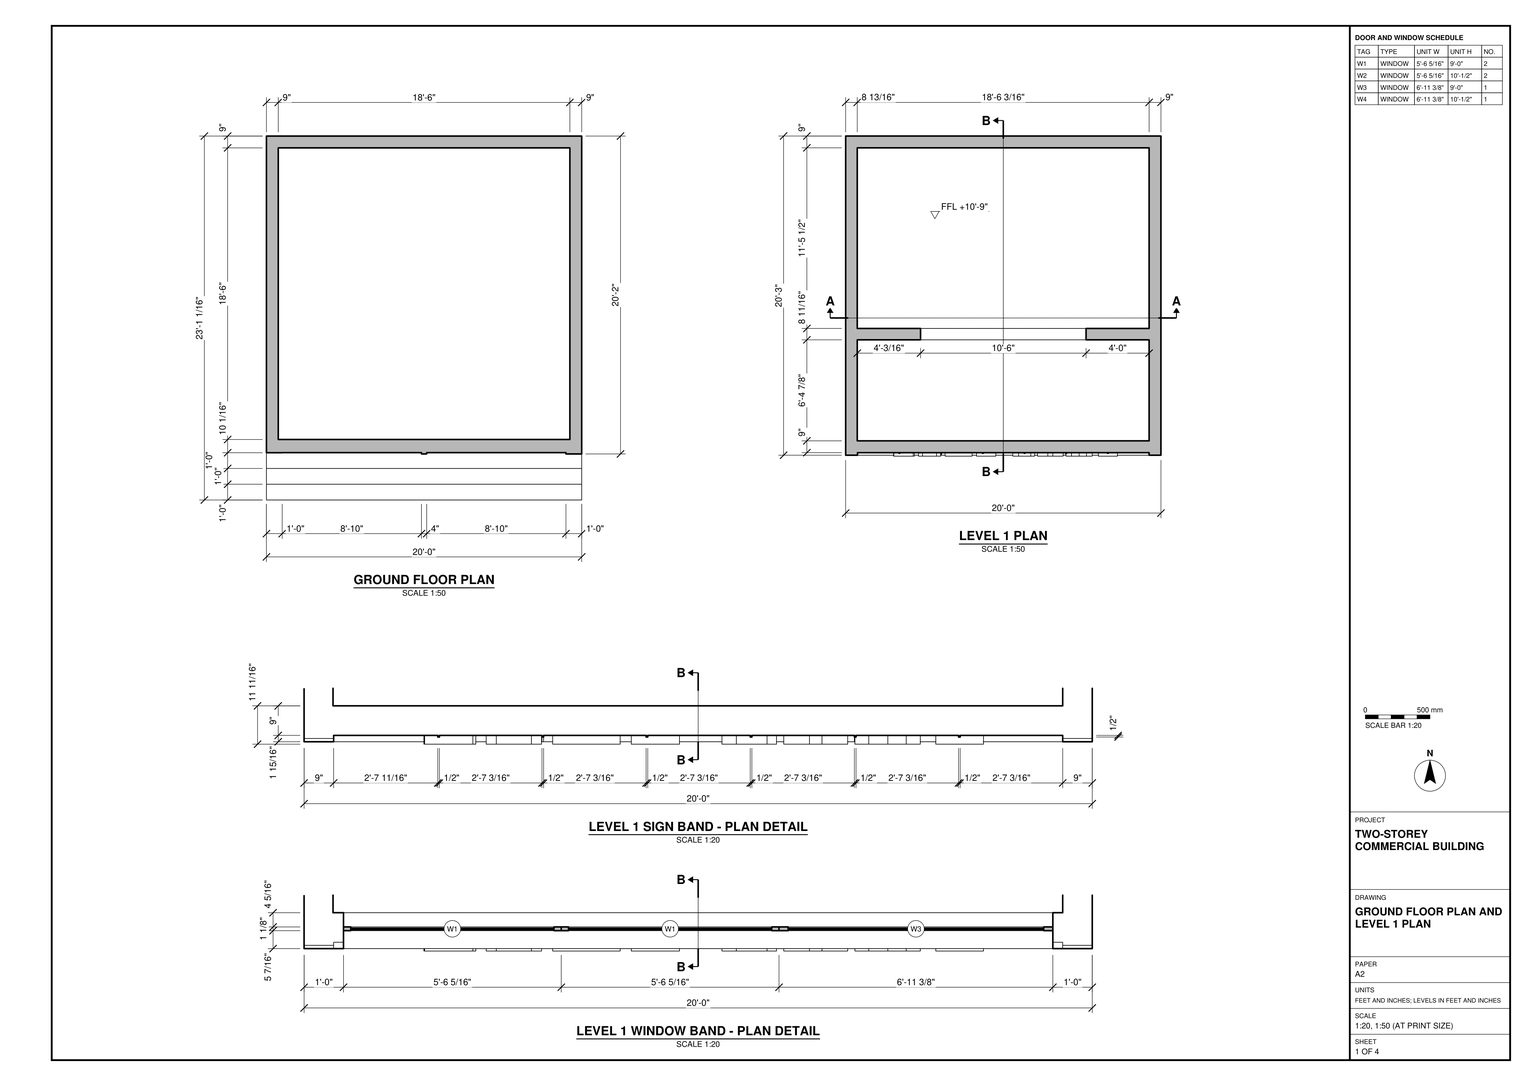
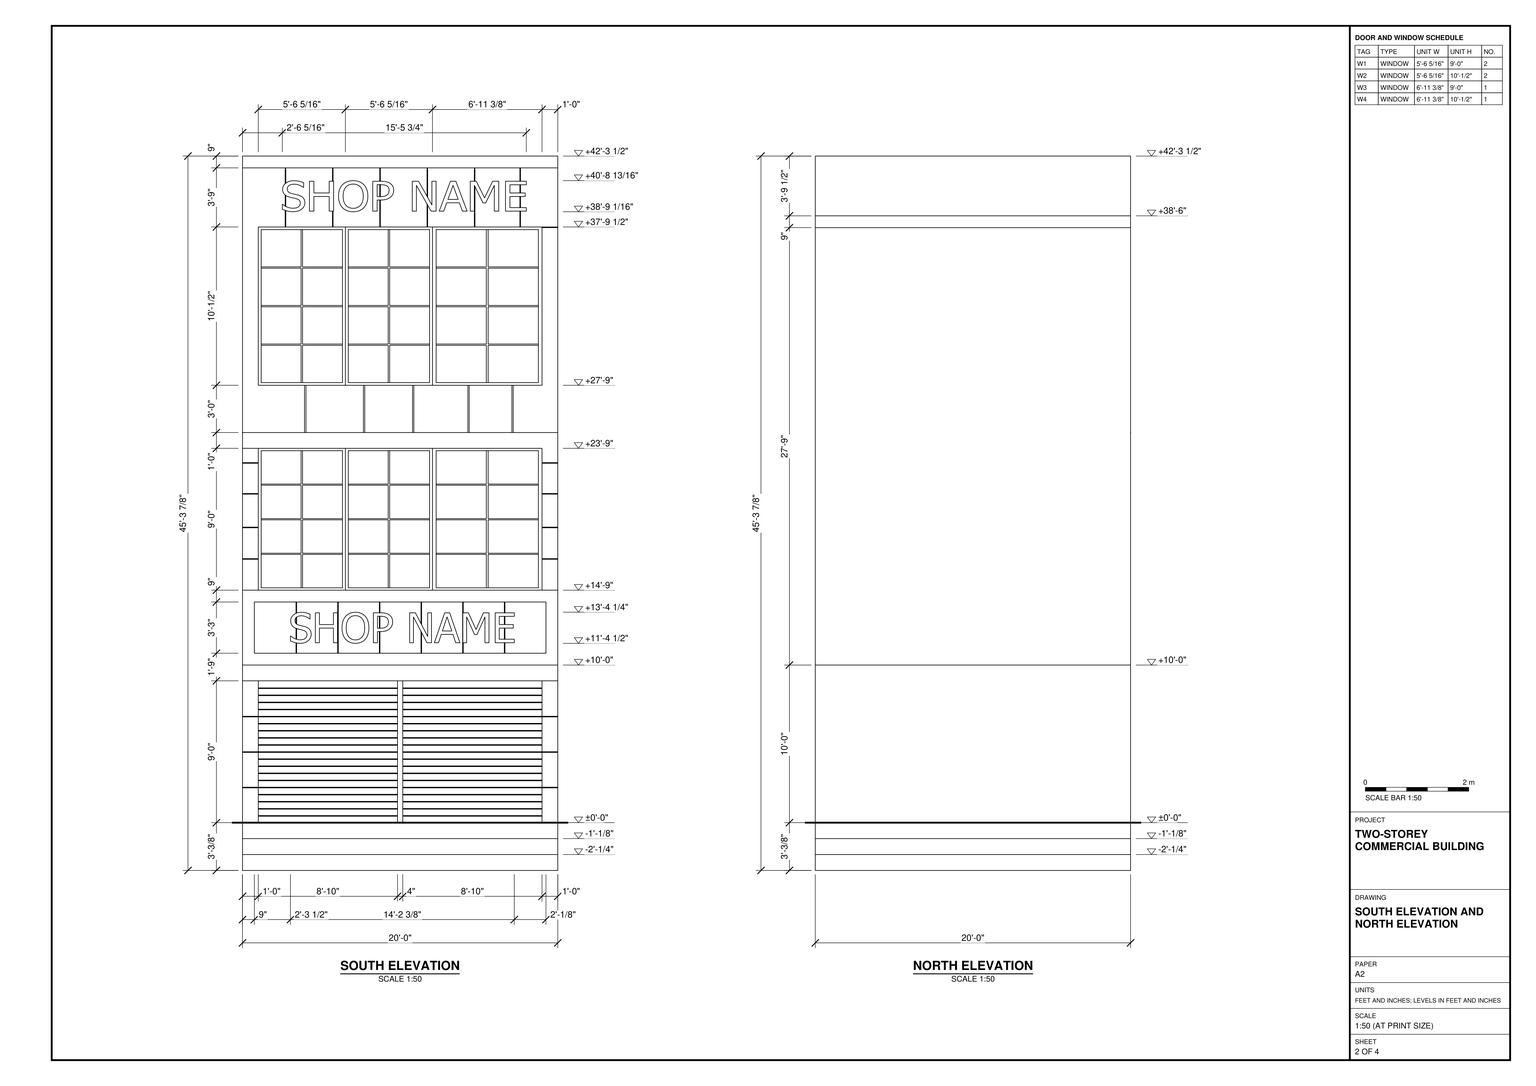
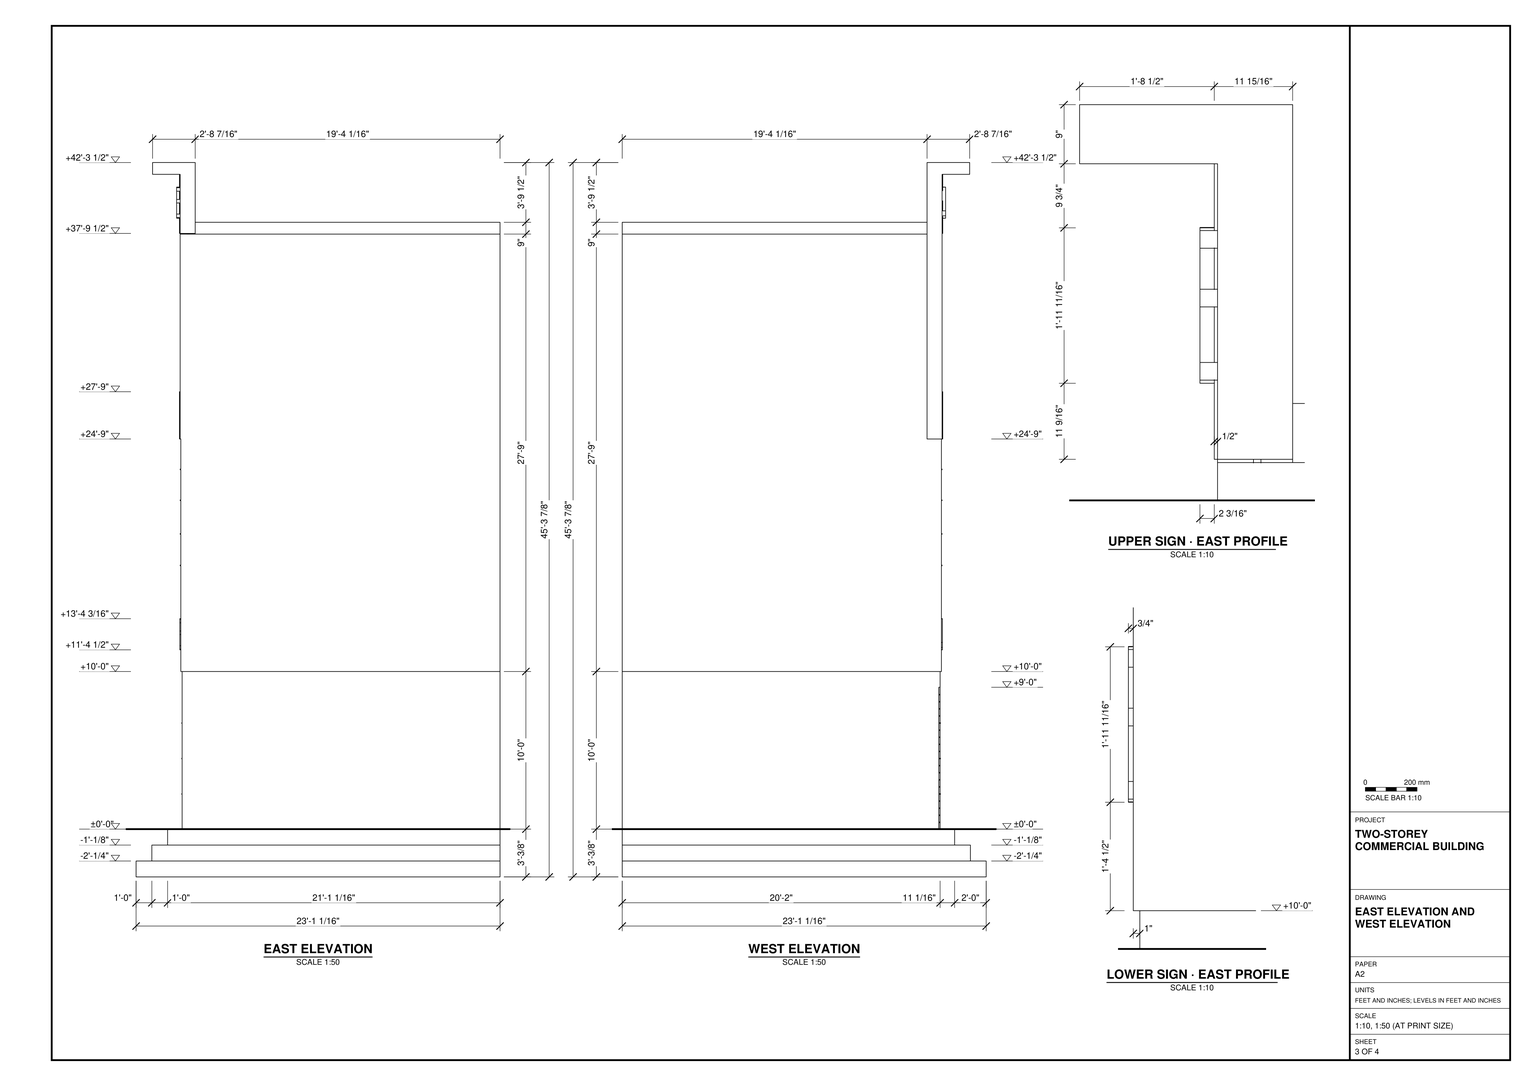
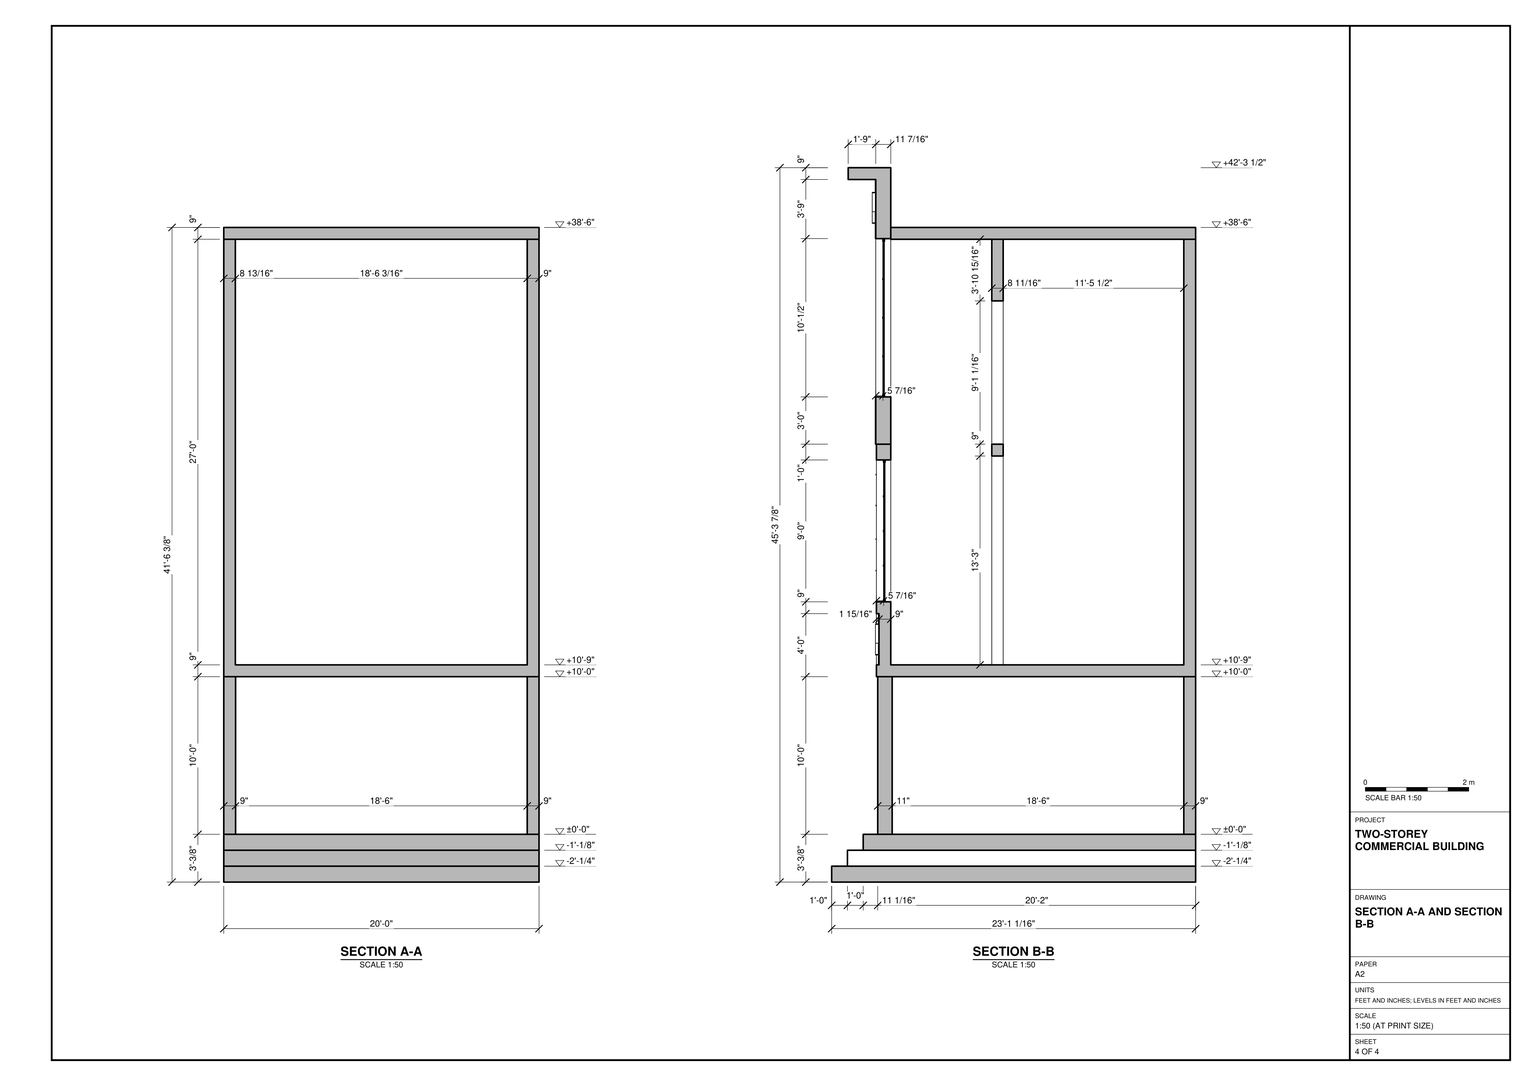
Build the two-storey commercial building in SketchUp from task_files/diagram_01.pdf. Work in feet and inches. Use the south elevation as the shopfront. The overall width is 20'-0", the depth is 23'-1 1/16", and the height is 45'-3 7/8", measured from the bottom of the stepped base to the top of the front cap. Set the ground-floor reference level at ±0'-0" and the level above at +10'-0".

Use the plans to lay out the rectangular shell, with the 9" ground-floor perimeter walls and the wall thicknesses shown on the upper plan. Include the floor slabs, the transverse wall with its broad central opening, and the flat roof slab behind the raised front sign. Keep the side and rear walls plain. Extend the entrance steps across the full shopfront width and model the two horizontally slatted shutter bays with their narrow central pier.

Above the shutters, build the lower sign band, two rows of framed windows separated by a solid band, and the upper sign band with its projecting cap. Follow the window divisions, sign-panel joints and lettering positions in the elevation and detail views.

Keep shell elements and any furniture or joinery pieces in separate groups or components, and use components for repeated parts. Any decor or loose items shown may use suitable library components. Save one SketchUp model as output_files/two_storey_shopfront_with_window_and_sign_bands.skp.

# SketchUp Ruby script. Lengths in inches.
U = 1.inch
M = Sketchup.active_model
def pt(a) = Geom::Point3d.new(a.map { |v| v * U })
def face(e, loops, mat)
  f = e.add_face(loops[0].map { |a| pt(a) })
  loops[1..].each { |l| e.add_face(l.map { |a| pt(a) }).erase! }
  f.material = f.back_material = mat if mat
  f
end
# faces: each face lists its corners as indices into pts; further lists are holes
def faces(e, pts, list, mat = nil) = list.each { |f| face(e, (f[0].is_a?(Array) ? f : [f]).map { |l| l.map { |i| pts[i] } }, mat) }
# xy, xz, yz: faces in a plane at the given z, y or x. An outline is a flat list of corners, or four numbers for a rectangle; further outlines are holes
def ring(l) = l.size == 4 ? [[l[0], l[1]], [l[2], l[1]], [l[2], l[3]], [l[0], l[3]]] : l.each_slice(2).to_a
def flat(e, list, mat, &to3) = list.each { |f| face(e, (f[0].is_a?(Array) ? f : [f]).map { |l| ring(l).map { |u, v| to3.(u, v) } }, mat) }
def xy(e, z, list, mat = nil) = flat(e, list, mat) { |x, y| [x, y, z] }
def xz(e, y, list, mat = nil) = flat(e, list, mat) { |x, z| [x, y, z] }
def yz(e, x, list, mat = nil) = flat(e, list, mat) { |y, z| [x, y, z] }
def lines(e, pts, list) = list.each { |a, b| e.add_line(pt(pts[a]), pt(pts[b])) }
# prism: a flat outline (further loops are holes) pulled along v
def prism(e, loops, v, mat = nil)
  f = face(e, loops, mat); d = Geom::Vector3d.new(v.map { |x| x * U })
  f.pushpull(f.normal.samedirection?(d) ? d.length : -d.length)
end
def box(e, o, s, mat = nil) = prism(e, [[o, [o[0] + s[0], o[1], o[2]], [o[0] + s[0], o[1] + s[1], o[2]], [o[0], o[1] + s[1], o[2]]]], [0, 0, s[2]], mat)
def at(x, y, z, deg = 0) = Geom::Transformation.translation(pt([x, y, z])) * Geom::Transformation.rotation(ORIGIN, Z_AXIS, deg.degrees)
def axes(o, x, y, z) = Geom::Transformation.new([*x, 0, *y, 0, *z, 0, *pt(o).to_a, 1])
def part(name) = M.definitions.add(name)
# library, detail: a bought-in or finely detailed component or shape, given as its bounding box
def library(name, o, s) = part(name).tap { |d| box(d.entities, o, s) }
def detail(e, o, s) = box(e.add_group.entities, o, s)
def put(e, d, t, mat = nil) = e.add_instance(d, t).tap { |i| i.material = mat if mat }
def group(e, t, mat = nil) = e.add_group.tap { |g| g.transformation = t; g.material = mat if mat }.entities
root = M.entities
M.materials.add("[0133_Gray]").color = [128, 128, 128]
M.materials.add("[0134_DimGray]").color = [163, 163, 163]
M.materials.add("[0134_DimGray]1").color = [105, 105, 105]
M.materials.add("[0135_DarkGray]").color = [71, 71, 71]
M.materials.add("[0135_DarkGray]1").color = [81, 81, 81]
M.materials.add("[0136_Charcoal]").color = [73, 73, 73]
M.materials.add("[Blinds Wood Light]").color = [155, 100, 14]
M.materials.add("[Translucent Glass Sky Reflection]").color = [163, 177, 193]
M.materials["[Translucent Glass Sky Reflection]"].alpha = 0.52
M.materials.add("[Wood Cherry Original]").color = [152, 86, 42]
M.materials.add("[Wood Floor Dark]").color = [153, 94, 42]
c1 = library("SHOP NAME",[0.49,0,0],[69.73,9.9,1])
c2 = part("WINDOW")
g1 = group(c2.entities,at(60,0,0))
g2 = group(g1,at(-2,0.5,2),"[Translucent Glass Sky Reflection]")
box(g2,[-56,0,0],[56,0.75,116])
g3 = group(g1,at(0,0,0))
xy(g3,0,[[-60,0,0,2]])
xy(g3,2,[[-58,0,-58,2,-2,2,-2,0,-29.5,0,-29.5,1.25,-30.5,1.25,-30.5,0]])
xy(g3,30.25,[[-58,0,-30.5,1.25],[-29.5,0,-2,1.25]])
xy(g3,31.25,[[-58,0,-30.5,1.25],[-29.5,0,-2,1.25]])
xy(g3,59.5,[[-58,0,-30.5,1.25],[-29.5,0,-2,1.25]])
xy(g3,60.5,[[-58,0,-30.5,1.25],[-29.5,0,-2,1.25]])
xy(g3,88.75,[[-58,0,-30.5,1.25],[-29.5,0,-2,1.25]])
xy(g3,89.75,[[-58,0,-30.5,1.25],[-29.5,0,-2,1.25]])
xy(g3,118,[[-58,0,-30.5,0,-30.5,1.25,-29.5,1.25,-29.5,0,-2,0,-2,2,-58,2]])
xy(g3,120,[[-60,0,0,2]])
xz(g3,0,[[[-60,0,0,120],[-58,2,-30.5,30.25],[-58,31.25,-30.5,59.5],[-29.5,2,-2,30.25],[-58,60.5,-30.5,88.75],[-58,89.75,-30.5,118],[-29.5,89.75,-2,118],[-29.5,60.5,-2,88.75],[-29.5,31.25,-2,59.5]]])
xz(g3,1.25,[[-30.5,2,-29.5,2,-29.5,30.25,-2,30.25,-2,31.25,-29.5,31.25,-29.5,59.5,-2,59.5,-2,60.5,-29.5,60.5,-29.5,88.75,-2,88.75,-2,89.75,-29.5,89.75,-29.5,118,-30.5,118,-30.5,89.75,-58,89.75,-58,88.75,-30.5,88.75,-30.5,60.5,-58,60.5,-58,59.5,-30.5,59.5,-30.5,31.25,-58,31.25,-58,30.25,-30.5,30.25]])
xz(g3,2,[[[-60,0,0,120],[-58,2,-2,118]]])
yz(g3,-60,[[0,0,2,120]])
yz(g3,-58,[[0,2,0,30.25,1.25,30.25,1.25,31.25,0,31.25,0,59.5,1.25,59.5,1.25,60.5,0,60.5,0,88.75,1.25,88.75,1.25,89.75,0,89.75,0,118,2,118,2,2]])
yz(g3,-30.5,[[0,2,1.25,30.25],[0,31.25,1.25,59.5],[0,60.5,1.25,88.75],[0,89.75,1.25,118]])
yz(g3,-29.5,[[0,2,1.25,30.25],[0,31.25,1.25,59.5],[0,60.5,1.25,88.75],[0,89.75,1.25,118]])
yz(g3,-2,[[0,2,2,2,2,118,0,118,0,89.75,1.25,89.75,1.25,88.75,0,88.75,0,60.5,1.25,60.5,1.25,59.5,0,59.5,0,31.25,1.25,31.25,1.25,30.25,0,30.25]])
yz(g3,0,[[0,0,2,120]])
p = [[-29.5,0,118],[-30.5,0,118]]
lines(g3,p,[[0,1]])
xy(root,0,[[[118,35.0625,118,36.0625,12,36.0625,12,36,0,36,0,277.0625,240,277.0625,240,35.0625,228,35.0625,228,36.0625,122,36.0625,122,35.0625],[9,46.0625,231,268.0625]],[9,46.0625,231,268.0625]])
xy(root,4.9,[[12,36.0625,118,37.0625],[122,36.0625,228,37.0625]])
xy(root,5.4,[[12,36.0625,118,37.0625],[122,36.0625,228,37.0625]])
xy(root,10.3,[[12,36.0625,118,37.0625],[122,36.0625,228,37.0625]])
xy(root,10.8,[[12,36.0625,118,37.0625],[122,36.0625,228,37.0625]])
xy(root,15.7,[[12,36.0625,118,37.0625],[122,36.0625,228,37.0625]])
xy(root,16.2,[[12,36.0625,118,37.0625],[122,36.0625,228,37.0625]])
xy(root,21.1,[[12,36.0625,118,37.0625],[122,36.0625,228,37.0625]])
xy(root,21.6,[[12,36.0625,118,37.0625],[122,36.0625,228,37.0625]])
xy(root,26.5,[[228,34.76,240,35.0625],[0,35.7,12,36],[12,36.0625,118,37.0625],[122,36.0625,228,37.0625]])
xy(root,27,[[228,34.76,240,35.0625],[0,35.7,12,36],[12,36.0625,118,37.0625],[122,36.0625,228,37.0625]])
xy(root,31.9,[[12,36.0625,118,37.0625],[122,36.0625,228,37.0625]])
xy(root,32.4,[[12,36.0625,118,37.0625],[122,36.0625,228,37.0625]])
xy(root,37.3,[[12,36.0625,118,37.0625],[122,36.0625,228,37.0625]])
xy(root,37.8,[[12,36,118,37.0625],[122,36.0625,228,37.0625]])
xy(root,42.7,[[12,36,118,37.0625],[122,36.0625,228,37.0625]])
xy(root,43.2,[[12,36.0625,118,37.0625],[122,36.0625,228,37.0625]])
xy(root,48.1,[[12,36.0625,118,37.0625],[122,36.0625,228,37.0625]])
xy(root,48.6,[[12,36.0625,118,37.0625],[122,36.0625,228,37.0625]])
xy(root,53.5,[[228,34.76,240,35.0625],[0,35.7,12,36],[12,36.0625,118,37.0625],[122,36.0625,228,37.0625]])
xy(root,54,[[228,34.76,240,35.0625],[0,35.7,12,36],[12,36.0625,118,37.0625],[122,36.0625,228,37.0625]])
xy(root,58.9,[[12,36.0625,118,37.0625],[122,36.0625,228,37.0625]])
xy(root,59.4,[[12,36.0625,118,37.0625],[122,36.0625,228,37.0625]])
xy(root,64.3,[[12,36.0625,118,37.0625],[122,36.0625,228,37.0625]])
xy(root,64.8,[[12,36.0625,118,37.0625],[122,36.0625,228,37.0625]])
xy(root,69.7,[[12,36.0625,118,37.0625],[122,36.0625,228,37.0625]])
xy(root,70.2,[[12,36.0625,118,37.0625],[122,36.0625,228,37.0625]])
xy(root,75.1,[[12,36.0625,118,37.0625],[122,36.0625,228,37.0625]])
xy(root,75.6,[[12,36.0625,118,37.0625],[122,36.0625,228,37.0625]])
xy(root,80.5,[[228,34.76,240,35.0625],[0,35.7,12,36],[12,36.0625,118,37.0625],[122,36.0625,228,37.0625]])
xy(root,81,[[228,34.76,240,35.0625],[0,35.7,12,36],[12,36.0625,118,37.0625],[122,36.0625,228,37.0625]])
xy(root,85.9,[[12,36.0625,118,37.0625],[122,36.0625,228,37.0625]])
xy(root,86.4,[[12,36.0625,118,37.0625],[122,36.0625,228,37.0625]])
xy(root,91.3,[[12,36.0625,118,37.0625],[122,36.0625,228,37.0625]])
xy(root,91.8,[[12,36.0625,118,37.0625],[122,36.0625,228,37.0625]])
xy(root,96.7,[[12,36.0625,118,37.0625],[122,36.0625,228,37.0625]])
xy(root,97.2,[[12,36.0625,118,37.0625],[122,36.0625,228,37.0625]])
xy(root,102.1,[[12,36.0625,118,37.0625],[122,36.0625,228,37.0625]])
xy(root,102.6,[[12,36.0625,118,37.0625],[122,36.0625,228,37.0625]])
xy(root,108,[[0,35.0625,12,36],[12,35.0625,118,36.0625],[122,35.0625,228,36.0625]])
xy(root,120,[[0,34.0625,240,35.0625],[0,35.0625,240,277.0625]])
xy(root,129,[[9,34.0625,40.71,36],[40.71,34.0625,41.21,35.5],[41.21,34.0625,72.43,36],[72.43,34.0625,72.93,35.5],[72.93,34.0625,104.14,36],
  [104.14,34.0625,104.64,35.5],[104.64,34.0625,135.86,36],[135.86,34.0625,136.36,35.5],[136.36,34.0625,167.57,36],[167.57,34.0625,168.07,35.5],
  [168.07,34.0625,199.29,36],[199.29,34.0625,199.79,35.5],[199.79,34.0625,231,36],[8.8125,45,231,121.9],[57,121.9,183,130.5625],
  [8.8125,130.5625,231,268.0625]])
xy(root,168,[[9,34.0625,40.71,36],[40.71,34.0625,41.21,35.5],[41.21,34.0625,72.43,36],[72.43,34.0625,72.93,35.5],[72.93,34.0625,104.14,36],
  [104.14,34.0625,104.64,35.5],[104.64,34.0625,135.86,36],[135.86,34.0625,136.36,35.5],[136.36,34.0625,167.57,36],[167.57,34.0625,168.07,35.5],
  [168.07,34.0625,199.29,36],[199.29,34.0625,199.79,35.5],[199.79,34.0625,231,36]])
xy(root,177,[[12,34.0625,228,45]])
xy(root,200.5,[[0,33.5625,12,34.0625],[228,33.5625,240,34.0625]])
xy(root,201,[[0,33.5625,12,34.0625],[228,33.5625,240,34.0625]])
xy(root,224.5,[[0,33.5625,12,34.0625],[228,33.5625,240,34.0625]])
xy(root,225,[[0,33.5625,12,34.0625],[228,33.5625,240,34.0625]])
xy(root,250.1,[[0,33.5625,12,34.0625],[228,33.5625,240,34.0625]])
xy(root,250.6,[[0,33.5625,12,34.0625],[228,33.5625,240,34.0625]])
xy(root,273.6,[[0,33.5625,12,34.0625],[228,33.5625,240,34.0625]])
xy(root,274.1,[[0,33.5625,12,34.0625],[228,33.5625,240,34.0625]])
xy(root,285,[[12,34.0625,228,45]])
xy(root,288,[[9,121.9,183,130.5625]])
xy(root,297,[[47.1875,33.0625,48.3125,34.0625],[92.0625,33.0625,93.0625,34.0625],[129.4375,33.0625,130.4375,34.0625],[171.5625,33.0625,172.5625,34.0625],[205.0625,33.0625,206.0625,34.0625],
  [0,33.5625,47.1875,34.0625],[48.3125,33.5625,92.0625,34.0625],[93.0625,33.5625,129.4375,34.0625],[130.4375,33.5625,171.5625,34.0625],[172.5625,33.5625,205.0625,34.0625],
  [206.0625,33.5625,231,34.0625],[231,33.5625,240,34.0625],[0,34.0625,231,45],[8.8125,121.9,9,130.5625],[57,121.9,183,130.5625]])
xy(root,333,[[47.1875,33.0625,48.3125,33.0625,48.3125,33.5625,92.0625,33.5625,92.0625,33.0625,93.0625,33.0625,93.0625,33.5625,129.4375,33.5625,129.4375,33.0625,130.4375,33.0625,130.4375,33.5625,171.5625,33.5625,171.5625,33.0625,172.5625,33.0625,172.5625,33.5625,205.0625,33.5625,205.0625,33.0625,206.0625,33.0625,206.0625,33.5625,228,33.5625,228,45,12,45,12,33.5625,47.1875,33.5625]])
xy(root,406.07,[[57,121.9,183,130.5625]])
xy(root,453,[[228,33.5625,240,45],[0,45,8.8125,277.0625],[8.8125,45,231,268.0625],[231,45,240,277.0625],[9,121.9,57,130.5625],
  [57,121.9,231,130.5625],[8.8125,268.0625,231,277.0625]])
xy(root,453.5,[[32.46,33.0625,32.46,33.5625,12,33.5625,12,45,240,45,240,33.5625,211.65,33.5625,211.65,33.0625,211.15,33.0625,211.15,33.5625,176.96,33.5625,176.96,33.0625,176.46,33.0625,176.46,33.5625,140.96,33.5625,140.96,33.0625,140.46,33.0625,140.46,33.5625,104.96,33.5625,104.96,33.0625,104.46,33.0625,104.46,33.5625,68.96,33.5625,68.96,33.0625,68.45,33.0625,68.45,33.5625,32.96,33.5625,32.96,33.0625]])
xy(root,462,[[0,45,240,277.0625]])
xy(root,498.5,[[0,12.5625,0,33.5625,32.46,33.5625,32.46,33.0625,32.96,33.0625,32.96,33.5625,68.45,33.5625,68.45,33.0625,68.96,33.0625,68.96,33.5625,104.46,33.5625,104.46,33.0625,104.96,33.0625,104.96,33.5625,140.46,33.5625,140.46,33.0625,140.96,33.0625,140.96,33.5625,176.46,33.5625,176.46,33.0625,176.96,33.0625,176.96,33.5625,211.15,33.5625,211.15,33.0625,211.65,33.0625,211.65,33.5625,240,33.5625,240,12.5625]],"[Wood Cherry Original]")
xy(root,507.5,[[0,12.5625,240,45]])
xz(root,12.5625,[[0,498.5,240,507.5]],"[0134_DimGray]1")
xz(root,33.0625,[[47.1875,297,48.3125,333],[92.0625,297,93.0625,333],[129.4375,297,130.4375,333],[171.5625,297,172.5625,333],[205.0625,297,206.0625,333],
  [32.46,453.5,32.96,498.5],[68.45,453.5,68.96,498.5],[104.46,453.5,104.96,498.5],[140.46,453.5,140.96,498.5],[176.46,453.5,176.96,498.5],
  [211.15,453.5,211.65,498.5]],"[0135_DarkGray]1")
xz(root,33.5625,[[228,200.5,240,201],[228,224.5,240,225],[228,250.1,240,250.6],[228,273.6,240,274.1],[140.46,498.5,140.96,507.5]])
xz(root,33.5625,[[0,297,47.1875,297,47.1875,333,12,333,12,453.5,32.46,453.5,32.46,498.5,0,498.5],[48.3125,297,92.0625,333],[93.0625,297,129.4375,333],[130.4375,297,171.5625,333],[172.5625,297,205.0625,333],
  [206.0625,297,240,297,240,453,228,453,228,333,206.0625,333],[32.96,453.5,68.45,498.5],[68.96,453.5,104.46,498.5],[104.96,453.5,140.46,498.5],[140.96,453.5,176.46,498.5],
  [176.96,453.5,211.15,498.5],[211.65,453.5,240,498.5]],"[0133_Gray]")
xz(root,33.5625,[[0,200.5,12,201],[0,224.5,12,225],[0,250.1,12,250.6],[0,273.6,12,274.1]],"[0135_DarkGray]1")
xz(root,34.0625,[[[0,120,240,177],[9,129,231,168]]])
xz(root,34.0625,[[0,177,12,200.5],[0,201,12,224.5],[0,225,12,250.1],[0,250.6,12,273.6],[0,274.1,12,285]],"[0133_Gray]")
xz(root,34.0625,[[228,177,240,200.5],[228,201,240,224.5],[228,225,240,250.1],[228,250.6,240,273.6],[228,274.1,240,274.1,240,297,0,297,0,285,228,285]],"[Wood Floor Dark]")
xz(root,34.76,[[228,26.5,240,27],[228,53.5,240,54],[228,80.5,240,81]],"[0134_DimGray]")
xz(root,35.0625,[[118,0,122,108],[228,0,240,26.5],[228,27,240,53.5],[228,54,240,80.5],[228,81,240,108]],"[0135_DarkGray]")
xz(root,35.0625,[[0,108,240,120]],"[Wood Floor Dark]")
xz(root,35.5,[[40.71,129,41.21,168],[72.43,129,72.93,168],[104.14,129,104.64,168],[135.86,129,136.36,168],[167.57,129,168.07,168],
  [199.29,129,199.79,168]],"[0133_Gray]")
xz(root,35.7,[[0,26.5,12,27],[0,53.5,12,54],[0,80.5,12,81]],"[0134_DimGray]")
xz(root,36,[[12,37.8,118,42.7]],"[0133_Gray]")
xz(root,36,[[0,0,12,26.5],[0,27,12,53.5],[0,54,12,80.5],[0,81,12,108],[9,129,40.71,168],
  [41.21,129,72.43,168],[72.93,129,104.14,168],[104.64,129,135.86,168],[136.36,129,167.57,168],[168.07,129,199.29,168],
  [199.79,129,231,168]],"[0135_DarkGray]")
xz(root,36.0625,[[12,0,118,4.9],[122,0,228,4.9],[12,5.4,118,10.3],[122,5.4,228,10.3],[12,10.8,118,15.7],
  [122,10.8,228,15.7],[12,16.2,118,21.1],[122,16.2,228,21.1],[12,21.6,118,26.5],[122,21.6,228,26.5],
  [12,27,118,31.9],[122,27,228,31.9],[12,32.4,118,37.3],[122,32.4,228,37.3],[122,37.8,228,42.7],
  [12,43.2,118,48.1],[122,43.2,228,48.1],[12,48.6,118,53.5],[122,48.6,228,53.5],[12,54,118,58.9],
  [122,54,228,58.9],[12,59.4,118,64.3],[122,59.4,228,64.3],[12,64.8,118,69.7],[122,64.8,228,69.7],
  [12,70.2,118,75.1],[122,70.2,228,75.1],[12,75.6,118,80.5],[122,75.6,228,80.5],[12,81,118,85.9],
  [122,81,228,85.9],[12,86.4,118,91.3],[122,86.4,228,91.3],[12,91.8,118,96.7],[122,91.8,228,96.7],
  [12,97.2,118,102.1],[122,97.2,228,102.1],[12,102.6,118,108],[122,102.6,228,108]],"[0133_Gray]")
xz(root,37.0625,[[12,4.9,118,5.4],[122,4.9,228,5.4],[12,10.3,118,10.8],[122,10.3,228,10.8],[12,15.7,118,16.2],
  [122,15.7,228,16.2],[12,21.1,118,21.6],[122,21.1,228,21.6],[12,26.5,118,27],[122,26.5,228,27],
  [12,31.9,118,32.4],[122,31.9,228,32.4],[12,37.3,118,37.8],[122,37.3,228,37.8],[12,42.7,118,43.2],
  [122,42.7,228,43.2],[12,48.1,118,48.6],[122,48.1,228,48.6],[12,53.5,118,54],[122,53.5,228,54],
  [12,58.9,118,59.4],[122,58.9,228,59.4],[12,64.3,118,64.8],[122,64.3,228,64.8],[12,69.7,118,70.2],
  [122,69.7,228,70.2],[12,75.1,118,75.6],[122,75.1,228,75.6],[12,80.5,118,81],[122,80.5,228,81],
  [12,85.9,118,86.4],[122,85.9,228,86.4],[12,91.3,118,91.8],[122,91.3,228,91.8],[12,96.7,118,97.2],
  [122,96.7,228,97.2],[12,102.1,118,102.6],[122,102.1,228,102.6]],"[0136_Charcoal]")
xz(root,45,[[8.8125,129,8.8125,297,231,297,231,285,12,285,12,177,231,177,231,129],[228,177,231,285],[0,297,8.8125,453],[8.8125,297,8.8125,453,12,453,12,333,228,333,228,453,231,453,231,297],[0,453,0,462,240,462,240,453.5,12,453.5,12,453],
  [12,453,240,453.5],[0,462,240,507.5]])
xz(root,46.0625,[[9,0,231,120]])
xz(root,121.9,[[8.8125,129,57,288],[183,129,231,129,231,453,57,453,57,406.07,183,406.07],[8.8125,288,9,297],[9,288,57,453],[57,288,183,297]])
xz(root,130.5625,[[8.8125,129,57,288],[183,129,183,288,57,288,57,297,183,297,183,406.07,57,406.07,57,453,231,453,231,129],[8.8125,288,9,297],[9,288,57,453]])
xz(root,268.0625,[[9,0,231,120],[8.8125,129,231,453]])
xz(root,277.0625,[[0,0,240,120],[0,120,240,453],[0,453,240,462]])
yz(root,0,[[36,0,36,26.5,35.7,26.5,35.7,27,36,27,36,53.5,35.7,53.5,35.7,54,36,54,36,80.5,35.7,80.5,35.7,81,36,81,36,108,35.0625,108,35.0625,120,277.0625,120,277.0625,0],[34.0625,120,34.0625,200.5,33.5625,200.5,33.5625,201,34.0625,201,34.0625,224.5,33.5625,224.5,33.5625,225,34.0625,225,34.0625,250.1,33.5625,250.1,33.5625,250.6,34.0625,250.6,34.0625,273.6,33.5625,273.6,33.5625,274.1,34.0625,274.1,34.0625,297,45,297,45,453,277.0625,453,277.0625,120],[33.5625,297,33.5625,498.5,12.5625,498.5,12.5625,507.5,45,507.5,45,297],[45,453,277.0625,462]])
yz(root,8.8125,[[45,129,121.9,129,121.9,297,130.5625,297,130.5625,129,268.0625,129,268.0625,453,45,453]])
yz(root,9,[[46.0625,0,268.0625,120],[34.0625,129,36,168],[121.9,288,130.5625,297],[121.9,297,130.5625,453]])
yz(root,12,[[36,0,36.0625,4.9],[36,4.9,37.0625,5.4],[36,5.4,36.0625,10.3],[36,10.3,37.0625,10.8],[36,10.8,36.0625,15.7],
  [36,15.7,37.0625,16.2],[36,16.2,36.0625,21.1],[36,21.1,37.0625,21.6],[36,21.6,36.0625,26.5],[35.7,26.5,37.0625,27],
  [36,27,36.0625,31.9],[36,31.9,37.0625,32.4],[36,32.4,36.0625,37.3],[36,37.3,37.0625,37.8],[36,42.7,37.0625,43.2],
  [36,43.2,36.0625,48.1],[36,48.1,37.0625,48.6],[36,48.6,36.0625,53.5],[35.7,53.5,37.0625,54],[36,54,36.0625,58.9],
  [36,58.9,37.0625,59.4],[36,59.4,36.0625,64.3],[36,64.3,37.0625,64.8],[36,64.8,36.0625,69.7],[36,69.7,37.0625,70.2],
  [36,70.2,36.0625,75.1],[36,75.1,37.0625,75.6],[36,75.6,36.0625,80.5],[35.7,80.5,37.0625,81],[36,81,36.0625,85.9],
  [36,85.9,37.0625,86.4],[36,86.4,36.0625,91.3],[36,91.3,37.0625,91.8],[36,91.8,36.0625,96.7],[36,96.7,37.0625,97.2],
  [36,97.2,36.0625,102.1],[36,102.1,37.0625,102.6],[36,102.6,36.0625,108],[34.0625,177,45,177,45,285,34.0625,285,34.0625,274.1,33.5625,274.1,33.5625,273.6,34.0625,273.6,34.0625,250.6,33.5625,250.6,33.5625,250.1,34.0625,250.1,34.0625,225,33.5625,225,33.5625,224.5,34.0625,224.5,34.0625,201,33.5625,201,33.5625,200.5,34.0625,200.5],[33.5625,333,45,453.5]])
yz(root,32.46,[[33.0625,453.5,33.5625,498.5]])
yz(root,32.96,[[33.0625,453.5,33.5625,498.5]])
yz(root,40.71,[[35.5,129,36,168]])
yz(root,41.21,[[35.5,129,36,168]])
yz(root,47.1875,[[33.0625,297,33.5625,333]])
yz(root,48.3125,[[33.0625,297,33.5625,333]])
yz(root,57,[[121.9,129,130.5625,297],[121.9,297,130.5625,406.07]])
yz(root,68.45,[[33.0625,453.5,33.5625,498.5]])
yz(root,68.96,[[33.0625,453.5,33.5625,498.5]])
yz(root,72.43,[[35.5,129,36,168]])
yz(root,72.93,[[35.5,129,36,168]])
yz(root,92.0625,[[33.0625,297,33.5625,333]])
yz(root,93.0625,[[33.0625,297,33.5625,333]])
yz(root,104.14,[[35.5,129,36,168]])
yz(root,104.46,[[33.0625,453.5,33.5625,498.5]])
yz(root,104.64,[[35.5,129,36,168]])
yz(root,104.96,[[33.0625,453.5,33.5625,498.5]])
yz(root,118,[[35.0625,4.9,37.0625,5.4],[35.0625,10.3,37.0625,10.8],[35.0625,15.7,37.0625,16.2],[35.0625,21.1,37.0625,21.6],[35.0625,26.5,37.0625,27],
  [35.0625,31.9,37.0625,32.4],[35.0625,37.3,37.0625,37.8],[35.0625,42.7,37.0625,43.2],[35.0625,48.1,37.0625,48.6],[35.0625,53.5,37.0625,54],
  [35.0625,58.9,37.0625,59.4],[35.0625,64.3,37.0625,64.8],[35.0625,69.7,37.0625,70.2],[35.0625,75.1,37.0625,75.6],[35.0625,80.5,37.0625,81],
  [35.0625,85.9,37.0625,86.4],[35.0625,91.3,37.0625,91.8],[35.0625,96.7,37.0625,97.2],[35.0625,102.1,37.0625,102.6]])
yz(root,118,[[35.0625,0,36.0625,4.9],[35.0625,5.4,36.0625,10.3],[35.0625,10.8,36.0625,15.7],[35.0625,16.2,36.0625,21.1],[35.0625,21.6,36.0625,26.5],
  [35.0625,27,36.0625,31.9],[35.0625,32.4,36.0625,37.3],[35.0625,37.8,36,42.7],[35.0625,43.2,36.0625,48.1],[35.0625,48.6,36.0625,53.5],
  [35.0625,54,36.0625,58.9],[35.0625,59.4,36.0625,64.3],[35.0625,64.8,36.0625,69.7],[35.0625,70.2,36.0625,75.1],[35.0625,75.6,36.0625,80.5],
  [35.0625,81,36.0625,85.9],[35.0625,86.4,36.0625,91.3],[35.0625,91.8,36.0625,96.7],[35.0625,97.2,36.0625,102.1],[35.0625,102.6,36.0625,108]],"[0135_DarkGray]")
yz(root,122,[[35.0625,4.9,37.0625,5.4],[35.0625,10.3,37.0625,10.8],[35.0625,15.7,37.0625,16.2],[35.0625,21.1,37.0625,21.6],[35.0625,26.5,37.0625,27],
  [35.0625,31.9,37.0625,32.4],[35.0625,37.3,37.0625,37.8],[35.0625,42.7,37.0625,43.2],[35.0625,48.1,37.0625,48.6],[35.0625,53.5,37.0625,54],
  [35.0625,58.9,37.0625,59.4],[35.0625,64.3,37.0625,64.8],[35.0625,69.7,37.0625,70.2],[35.0625,75.1,37.0625,75.6],[35.0625,80.5,37.0625,81],
  [35.0625,85.9,37.0625,86.4],[35.0625,91.3,37.0625,91.8],[35.0625,96.7,37.0625,97.2],[35.0625,102.1,37.0625,102.6]])
yz(root,122,[[35.0625,0,36.0625,4.9],[35.0625,5.4,36.0625,10.3],[35.0625,10.8,36.0625,15.7],[35.0625,16.2,36.0625,21.1],[35.0625,21.6,36.0625,26.5],
  [35.0625,27,36.0625,31.9],[35.0625,32.4,36.0625,37.3],[35.0625,37.8,36.0625,42.7],[35.0625,43.2,36.0625,48.1],[35.0625,48.6,36.0625,53.5],
  [35.0625,54,36.0625,58.9],[35.0625,59.4,36.0625,64.3],[35.0625,64.8,36.0625,69.7],[35.0625,70.2,36.0625,75.1],[35.0625,75.6,36.0625,80.5],
  [35.0625,81,36.0625,85.9],[35.0625,86.4,36.0625,91.3],[35.0625,91.8,36.0625,96.7],[35.0625,97.2,36.0625,102.1],[35.0625,102.6,36.0625,108]],"[0135_DarkGray]")
yz(root,129.4375,[[33.0625,297,33.5625,333]])
yz(root,130.4375,[[33.0625,297,33.5625,333]])
yz(root,135.86,[[35.5,129,36,168]])
yz(root,136.36,[[35.5,129,36,168]])
yz(root,140.46,[[33.0625,453.5,33.5625,498.5]])
yz(root,140.96,[[33.0625,453.5,33.5625,498.5]])
yz(root,167.57,[[35.5,129,36,168]])
yz(root,168.07,[[35.5,129,36,168]])
yz(root,171.5625,[[33.0625,297,33.5625,333]])
yz(root,172.5625,[[33.0625,297,33.5625,333]])
yz(root,176.46,[[33.0625,453.5,33.5625,498.5]])
yz(root,176.96,[[33.0625,453.5,33.5625,498.5]])
yz(root,183,[[121.9,129,130.5625,288],[121.9,297,130.5625,406.07]])
yz(root,199.29,[[35.5,129,36,168]])
yz(root,199.79,[[35.5,129,36,168]])
yz(root,205.0625,[[33.0625,297,33.5625,333]])
yz(root,206.0625,[[33.0625,297,33.5625,333]])
yz(root,211.15,[[33.0625,453.5,33.5625,498.5]])
yz(root,211.65,[[33.0625,453.5,33.5625,498.5]])
yz(root,228,[[35.0625,0,35.0625,5.4,37.0625,5.4,37.0625,4.9,36.0625,4.9,36.0625,0],[35.0625,5.4,35.0625,10.8,37.0625,10.8,37.0625,10.3,36.0625,10.3,36.0625,5.4],[35.0625,10.8,35.0625,16.2,37.0625,16.2,37.0625,15.7,36.0625,15.7,36.0625,10.8],[35.0625,16.2,35.0625,21.6,37.0625,21.6,37.0625,21.1,36.0625,21.1,36.0625,16.2],[35.0625,21.6,35.0625,26.5,34.76,26.5,34.76,27,37.0625,27,37.0625,26.5,36.0625,26.5,36.0625,21.6],
  [35.0625,27,35.0625,32.4,37.0625,32.4,37.0625,31.9,36.0625,31.9,36.0625,27],[35.0625,32.4,35.0625,37.8,37.0625,37.8,37.0625,37.3,36.0625,37.3,36.0625,32.4],[35.0625,37.8,35.0625,43.2,37.0625,43.2,37.0625,42.7,36.0625,42.7,36.0625,37.8],[35.0625,43.2,35.0625,48.6,37.0625,48.6,37.0625,48.1,36.0625,48.1,36.0625,43.2],[35.0625,48.6,35.0625,53.5,34.76,53.5,34.76,54,37.0625,54,37.0625,53.5,36.0625,53.5,36.0625,48.6],
  [35.0625,54,35.0625,59.4,37.0625,59.4,37.0625,58.9,36.0625,58.9,36.0625,54],[35.0625,59.4,35.0625,64.8,37.0625,64.8,37.0625,64.3,36.0625,64.3,36.0625,59.4],[35.0625,64.8,35.0625,70.2,37.0625,70.2,37.0625,69.7,36.0625,69.7,36.0625,64.8],[35.0625,70.2,35.0625,75.6,37.0625,75.6,37.0625,75.1,36.0625,75.1,36.0625,70.2],[35.0625,75.6,35.0625,80.5,34.76,80.5,34.76,81,37.0625,81,37.0625,80.5,36.0625,80.5,36.0625,75.6],
  [35.0625,81,35.0625,86.4,37.0625,86.4,37.0625,85.9,36.0625,85.9,36.0625,81],[35.0625,86.4,35.0625,91.8,37.0625,91.8,37.0625,91.3,36.0625,91.3,36.0625,86.4],[35.0625,91.8,35.0625,97.2,37.0625,97.2,37.0625,96.7,36.0625,96.7,36.0625,91.8],[35.0625,97.2,35.0625,102.6,37.0625,102.6,37.0625,102.1,36.0625,102.1,36.0625,97.2],[35.0625,102.6,36.0625,108],
  [34.0625,177,34.0625,200.5,33.5625,200.5,33.5625,201,34.0625,201,34.0625,224.5,33.5625,224.5,33.5625,225,34.0625,225,34.0625,250.1,33.5625,250.1,33.5625,250.6,34.0625,250.6,34.0625,273.6,33.5625,273.6,33.5625,274.1,34.0625,274.1,34.0625,285,45,285,45,177],[33.5625,333,45,453]])
yz(root,231,[[46.0625,0,268.0625,120],[34.0625,129,36,168],[45,129,121.9,453],[130.5625,129,268.0625,453]])
yz(root,240,[[35.0625,0,277.0625,0,277.0625,120,35.0625,120,35.0625,81,34.76,81,34.76,80.5,35.0625,80.5,35.0625,54,34.76,54,34.76,53.5,35.0625,53.5,35.0625,27,34.76,27,34.76,26.5,35.0625,26.5],[34.0625,120,277.0625,120,277.0625,453,33.5625,453,33.5625,297,34.0625,297,34.0625,274.1,33.5625,274.1,33.5625,273.6,34.0625,273.6,34.0625,250.6,33.5625,250.6,33.5625,250.1,34.0625,250.1,34.0625,225,33.5625,225,33.5625,224.5,34.0625,224.5,34.0625,201,33.5625,201,33.5625,200.5,34.0625,200.5],[45,453,277.0625,462],[33.5625,453.5,45,453.5,45,507.5,12.5625,507.5,12.5625,498.5,33.5625,498.5]])
p = [[32.96,33.5625,507.5],[32.96,33.5625,498.5],[176.46,33.5625,507.5],[176.46,33.5625,498.5],[32.46,33.5625,498.5],[32.46,33.5625,507.5],
  [68.45,33.5625,498.5],[68.45,33.5625,507.5],[104.46,33.5625,498.5],[104.46,33.5625,507.5],[68.96,33.5625,498.5],[104.96,33.5625,498.5],
  [176.96,33.5625,498.5],[211.65,33.5625,498.5],[211.15,33.5625,498.5],[8.8125,130.5625,297],[-0.1875,130.5625,297]]
lines(root,p,[[0,1],[2,3],[4,5],[6,7],[8,9],[1,4],[10,6],[11,8],[12,3],[13,14],[15,16]])
put(root,c1,axes([35.28,36,136.51],[2.4436,0,0],[0,0,2.3956],[0,-2.68,0]))
put(root,c1,axes([28.99,33.5625,465.08],[2.66352,0,0],[0,0,2.3956],[0,-2.68,0]))
put(root,c2,axes([12,39.53,177],[1.10512,0,0],[0,0.57,0],[0,0,0.9]))
put(root,c2,axes([78.31,39.53,177],[1.10512,0,0],[0,0.57,0],[0,0,0.9]))
put(root,c2,axes([144.61,39.53,177],[1.38977,0,0],[0,0.57,0],[0,0,0.9]))
put(root,c2,axes([144.61,39.03,333],[1.38977,0,0],[0,0.57,0],[0,0,1.00417]))
put(root,c2,axes([12,39.03,333],[1.10512,0,0],[0,0.57,0],[0,0,1.00417]))
put(root,c2,axes([78.31,39.03,333],[1.10512,0,0],[0,0.57,0],[0,0,1.00417]))
g4 = group(root,at(0,24,-12.125),"[0134_DimGray]1")
xy(g4,0,[[0,0,240,253.0625]])
xy(g4,12.125,[[0,0,240,253.0625]])
xz(g4,0,[[0,0,240,12.125]],"[Blinds Wood Light]")
xz(g4,253.0625,[[0,0,240,12.125]])
yz(g4,0,[[0,0,253.0625,12.125]])
yz(g4,240,[[0,0,253.0625,12.125]])
g5 = group(root,at(0,12,-24.25),"[0134_DimGray]1")
xy(g5,0,[[0,0,240,265.0625]])
xy(g5,12.125,[[0,0,240,265.0625]])
xz(g5,0,[[0,0,240,12.125]],"[Blinds Wood Light]")
xz(g5,265.0625,[[0,0,240,12.125]])
yz(g5,0,[[0,0,265.0625,12.125]])
yz(g5,240,[[0,0,265.0625,12.125]])
g6 = group(root,at(0,0,-36.375),"[0134_DimGray]1")
xy(g6,0,[[0,0,240,277.0625]])
xy(g6,12.125,[[0,0,240,277.0625]])
xz(g6,0,[[0,0,240,12.125]],"[Blinds Wood Light]")
xz(g6,277.0625,[[0,0,240,12.125]])
yz(g6,0,[[0,0,277.0625,12.125]])
yz(g6,240,[[0,0,277.0625,12.125]])
